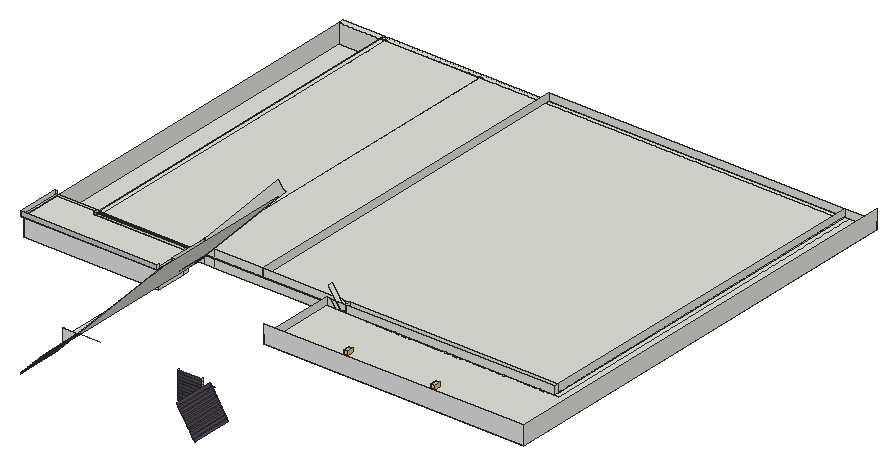
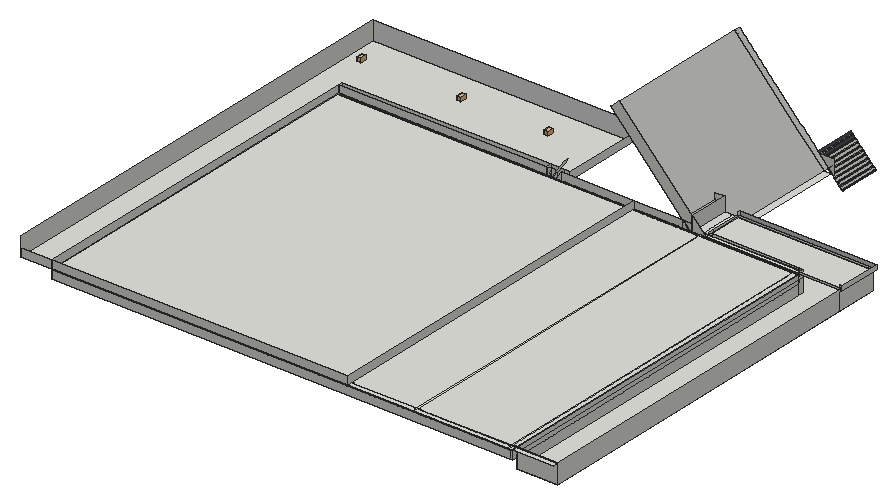
# SketchUp Ruby script. Lengths in inches.
U = 1.inch
M = Sketchup.active_model
def pt(a) = Geom::Point3d.new(a.map { |v| v * U })
def face(e, loops, mat)
  f = e.add_face(loops[0].map { |a| pt(a) })
  loops[1..].each { |l| e.add_face(l.map { |a| pt(a) }).erase! }
  f.material = f.back_material = mat if mat
  f
end
# faces: each face lists its corners as indices into pts; further lists are holes
def faces(e, pts, list, mat = nil) = list.each { |f| face(e, (f[0].is_a?(Array) ? f : [f]).map { |l| l.map { |i| pts[i] } }, mat) }
# xy, xz, yz: faces in a plane at the given z, y or x. An outline is a flat list of corners, or four numbers for a rectangle; further outlines are holes
def ring(l) = l.size == 4 ? [[l[0], l[1]], [l[2], l[1]], [l[2], l[3]], [l[0], l[3]]] : l.each_slice(2).to_a
def flat(e, list, mat, &to3) = list.each { |f| face(e, (f[0].is_a?(Array) ? f : [f]).map { |l| ring(l).map { |u, v| to3.(u, v) } }, mat) }
def xy(e, z, list, mat = nil) = flat(e, list, mat) { |x, y| [x, y, z] }
def xz(e, y, list, mat = nil) = flat(e, list, mat) { |x, z| [x, y, z] }
def yz(e, x, list, mat = nil) = flat(e, list, mat) { |y, z| [x, y, z] }
def lines(e, pts, list) = list.each { |a, b| e.add_line(pt(pts[a]), pt(pts[b])) }
# prism: a flat outline (further loops are holes) pulled along v
def prism(e, loops, v, mat = nil)
  f = face(e, loops, mat); d = Geom::Vector3d.new(v.map { |x| x * U })
  f.pushpull(f.normal.samedirection?(d) ? d.length : -d.length)
end
def box(e, o, s, mat = nil) = prism(e, [[o, [o[0] + s[0], o[1], o[2]], [o[0] + s[0], o[1] + s[1], o[2]], [o[0], o[1] + s[1], o[2]]]], [0, 0, s[2]], mat)
def at(x, y, z, deg = 0) = Geom::Transformation.translation(pt([x, y, z])) * Geom::Transformation.rotation(ORIGIN, Z_AXIS, deg.degrees)
def axes(o, x, y, z) = Geom::Transformation.new([*x, 0, *y, 0, *z, 0, *pt(o).to_a, 1])
def part(name) = M.definitions.add(name)
# library, detail: a bought-in or finely detailed component or shape, given as its bounding box
def library(name, o, s) = part(name).tap { |d| box(d.entities, o, s) }
def detail(e, o, s) = box(e.add_group.entities, o, s)
def put(e, d, t, mat = nil) = e.add_instance(d, t).tap { |i| i.material = mat if mat }
def group(e, t, mat = nil) = e.add_group.tap { |g| g.transformation = t; g.material = mat if mat }.entities
root = M.entities
M.materials.add("[Color M01]").color = [226, 226, 226]
M.materials.add("[Color M02]").color = [198, 198, 198]
M.materials.add("[Color M06]").color = [79, 71, 84]
c1 = library("Group\#13",[0,0,0],[3.54,3.54,3.9375])
xy(root,306.39,[[1096.79,2375.74,1127.76,2378.12]])
xy(root,307.2,[[1096.79,2375.74,1127.76,2378.12]])
xy(root,310.33,[[1096.79,2375.74,1127.76,2378.12]])
xy(root,311.14,[[1096.79,2375.74,1127.76,2378.12]])
xy(root,314.27,[[1096.79,2375.74,1127.76,2378.12]])
xy(root,315.08,[[1096.79,2376.24,1127.76,2378.12]])
xy(root,315.25,[[771.375,2530.63,771.375,3047.67,824.9375,3047.67,824.9375,2578.12,948.3125,2578.12,948.3125,2530.63]])
xy(root,318.2,[[1096.79,2376.24,1127.76,2378.12]])
xy(root,319.01,[[1096.79,2376.24,1127.76,2378.12]])
xy(root,322.14,[[1096.79,2376.24,1127.76,2378.12]])
xy(root,322.89,[[1096.79,2376.24,1127.76,2378.12]])
xy(root,326.02,[[1096.79,2376.24,1127.76,2378.12]])
xy(root,326.08,[[946.73,2380.48,955.23,2571.2],[946.73,2571.2,955.23,2571.59]])
xy(root,326.76,[[1096.79,2376.24,1127.76,2378.12]])
xy(root,328,[[824.9375,2584.2,1429.3,3053.87]])
xy(root,329.89,[[1096.79,2376.24,1127.76,2378.12]])
xy(root,330.64,[[1096.79,2376.24,1127.76,2378.12]])
xy(root,333.125,[[824.9375,2578.12,828.75,2584.2],[824.9375,2584.2,828.75,2586.43],[824.9375,2586.43,828.75,3047.67]])
xy(root,333.77,[[1096.79,2376.24,1127.76,2378.12]])
xy(root,334.51,[[1096.79,2376.24,1127.76,2378.12]])
xy(root,337.64,[[1096.79,2376.24,1127.76,2378.12]])
xy(root,338.39,[[1096.79,2376.24,1127.76,2378.12]])
xy(root,338.875,[[824.9375,2584.2,1429.3,3053.87]])
xy(root,340.125,[[1130.09,2475.84,1130.09,2578.12,1182.42,2578.12,1182.42,2576.81,1188.5,2576.81,1188.5,2578.12,1191.92,2578.12,1191.92,2576.81,1198,2576.81,1198,2578.12,1201.42,2578.12,1201.42,2576.81,1207.5,2576.81,1207.5,2578.12,1210.92,2578.12,1210.92,2576.81,1217,2576.81,1217,2578.12,1220.42,2578.12,1220.42,2576.81,1226.5,2576.81,1226.5,2578.12,1229.92,2578.12,1229.92,2576.81,1236,2576.81,1236,2578.12,1239.42,2578.12,1239.42,2576.81,1245.5,2576.81,1245.5,2578.12,1248.92,2578.12,1248.92,2576.81,1255,2576.81,1255,2578.12,1258.42,2578.12,1258.42,2576.81,1264.5,2576.81,1264.5,2578.12,1267.92,2578.12,1267.92,2576.81,1274,2576.81,1274,2578.12,1277.42,2578.12,1277.42,2576.81,1283.5,2576.81,1283.5,2578.12,1286.92,2578.12,1286.92,2576.81,1293,2576.81,1293,2578.12,1296.42,2578.12,1296.42,2576.81,1302.5,2576.81,1302.5,2578.12,1305.92,2578.12,1305.92,2576.81,1312,2576.81,1312,2578.12,1315.42,2578.12,1315.42,2576.81,1321.5,2576.81,1321.5,2578.12,1324.92,2578.12,1324.92,2576.81,1331,2576.81,1331,2578.12,1334.42,2578.12,1334.42,2576.81,1340.5,2576.81,1340.5,2578.12,1343.92,2578.12,1343.92,2576.81,1350,2576.81,1350,2578.12,1353.42,2578.12,1353.42,2576.81,1359.5,2576.81,1359.5,2578.12,1362.92,2578.12,1362.92,2576.81,1369,2576.81,1369,2578.12,1372.42,2578.12,1372.42,2576.81,1378.5,2576.81,1378.5,2578.12,1381.92,2578.12,1381.92,2576.81,1388,2576.81,1388,2578.12,1391.42,2578.12,1391.42,2576.81,1397.5,2576.81,1397.5,2578.12,1400.92,2578.12,1400.92,2576.81,1407,2576.81,1407,2578.12,1410.42,2578.12,1410.42,2576.81,1416.5,2576.81,1416.5,2578.12,1419.92,2578.12,1419.92,2576.81,1426,2576.81,1426,2578.12,1429.42,2578.12,1429.42,2576.81,1435.5,2576.81,1435.5,3053.87,1470.74,3053.87,1470.74,2475.84],[768.8125,2528.07,771.375,2530.63],[771.375,2528.07,948.3125,2530.63],[768.8125,2530.63,771.375,2584.2],[771.375,2530.63,771.375,2584.2,824.9375,2584.2,824.9375,2578.12,948.3125,2578.12,948.3125,2530.63],
  [948.3125,2530.63,954.51,2578.12],[954.51,2530.63,955.23,2578.12],[955.23,2530.63,965.61,2578.12],[965.61,2530.63,968.45,2578.12],[1182.42,2576.81,1188.5,2578.12],
  [1191.92,2576.81,1198,2578.12],[1201.42,2576.81,1207.5,2578.12],[1210.92,2576.81,1217,2578.12],[1220.42,2576.81,1226.5,2578.12],[1229.92,2576.81,1236,2578.12],
  [1239.42,2576.81,1245.5,2578.12],[1248.92,2576.81,1255,2578.12],[1258.42,2576.81,1264.5,2578.12],[1267.92,2576.81,1274,2578.12],[1277.42,2576.81,1283.5,2578.12],
  [1286.92,2576.81,1293,2578.12],[1296.42,2576.81,1302.5,2578.12],[1305.92,2576.81,1312,2578.12],[1315.42,2576.81,1321.5,2578.12],[1324.92,2576.81,1331,2578.12],
  [1334.42,2576.81,1340.5,2578.12],[1343.92,2576.81,1350,2578.12],[1353.42,2576.81,1359.5,2578.12],[1362.92,2576.81,1369,2578.12],[1372.42,2576.81,1378.5,2578.12],
  [1381.92,2576.81,1388,2578.12],[1391.42,2576.81,1397.5,2578.12],[1400.92,2576.81,1407,2578.12],[1410.42,2576.81,1416.5,2578.12],[1419.92,2576.81,1426,2578.12],
  [1429.42,2576.81,1435.5,3053.87],[824.9375,2578.12,831.01,2584.2],[831.01,2578.12,954.51,2584.2],[955.23,2578.12,965.61,2584.2],[965.61,2578.12,968.45,2584.2],
  [1156.15,2578.12,1429.3,2584.2],[1429.3,2578.12,1429.42,2584.2],[824.9375,2584.2,831.01,2586.43],[831.01,2584.2,954.51,2584.2,954.51,2584.32,831.14,2584.32,831.14,2586.43,831.01,2586.43],[954.51,2584.2,955.23,2586.43],
  [955.23,2584.2,1041.36,2586.43],[1041.36,2584.2,1156.15,2586.43],[1156.15,2584.2,1429.3,2586.43],[1429.3,2584.2,1429.42,2586.43],[831.14,2584.32,954.51,2586.43],
  [824.9375,2586.43,831.01,3047.67],[831.01,2586.43,831.14,3047.67],[831.14,2586.43,954.51,3047.67],[954.51,2586.43,955.23,3047.67],[955.23,2586.43,1041.36,3047.67],
  [1041.36,2586.43,1429.3,3047.67],[1429.3,2586.43,1429.42,3047.79],[771.375,3047.67,824.9375,3047.79],[824.9375,3047.67,828.75,3047.79],[828.75,3047.67,831.01,3047.79],
  [831.01,3047.67,954.51,3047.79],[954.51,3047.67,955.23,3047.79],[955.23,3047.67,1041.36,3047.79],[1041.36,3047.67,1429.3,3047.79],[771.375,3047.79,824.9375,3053.87],
  [824.9375,3047.79,828.75,3053.87],[828.75,3047.79,831.01,3053.87],[831.01,3047.79,954.51,3053.87],[954.51,3047.79,955.23,3053.87],[955.23,3047.79,1041.36,3053.87],
  [1041.36,3047.79,1429.3,3053.87],[1429.3,3047.79,1429.42,3053.87]])
xz(root,2373.56,[[1164.8,305.32,1165.17,305.56,1163.47,308.2,1163.11,307.97],[937.8,306.65,937.35,307.08,939.77,309.65,940.22,309.22],[937.35,307.08,937.12,307.29,939.54,309.87,939.77,309.65],[1162.57,308.8,1162.94,309.03,1161.25,311.68,1160.88,311.44],[941.1,310.16,940.64,310.59,943.07,313.16,943.52,312.73],
  [1160.35,312.27,1160.72,312.51,1159.02,315.15,1158.65,314.91],[944.4,313.66,943.94,314.09,946.36,316.66,946.82,316.23],[1158.12,315.74,1158.49,315.98,1156.8,318.62,1156.43,318.38],[947.7,317.17,947.24,317.59,948.3125,318.73,948.3125,317.82],[948.3125,317.82,948.77,318.3,948.3125,318.73],
  [948.77,318.3,950.12,319.74,949.66,320.17,948.3125,318.73],[948.3125,318.73,949.66,320.17,950.54,321.1,952.96,323.67,953.84,324.6,955.23,326.08,956.26,327.17,957.14,328.11,959.56,330.68,960.4375,331.61,962.86,334.18,963.73,335.11,966.16,337.6875,967.03,338.62,968.45,340.125,948.3125,340.125],[1155.9,319.21,1156.26,319.45,1154.57,322.09,1154.2,321.86],[951,320.67,953.42,323.24,952.96,323.67,950.54,321.1],[1153.67,322.6875,1154.04,322.92,1152.34,325.57,1151.98,325.33],
  [954.29,324.17,953.84,324.6,955.23,326.08,955.23,325.17],[955.23,325.17,955.6875,325.65,955.23,326.08],[955.6875,325.65,956.71,326.75,956.26,327.17,955.23,326.08],[1151.44,326.16,1151.8125,326.4,1150.12,329.04,1149.75,328.8],[957.59,327.68,960.01,330.25,959.56,330.68,957.14,328.11],
  [1149.22,329.63,1149.59,329.87,1147.89,332.51,1147.52,332.28],[960.89,331.18,963.3125,333.75,962.86,334.18,960.4375,331.61],[1146.99,333.11,1147.36,333.34,1145.66,335.98,1145.3,335.75],[964.1875,334.6875,966.61,337.26,966.16,337.6875,963.73,335.11],[1144.76,336.58,1145.13,336.8125,1143.4375,339.46,1143.07,339.22],
  [967.49,338.19,968.91,339.7,968.45,340.125,967.03,338.62],[968.91,339.7,969.31,340.125,968.45,340.125],[1142.54,340.05,1142.91,340.29,1141.21,342.93,1140.84,342.69],[968.45,340.125,969.31,340.125,969.91,340.76,969.45,341.19]])
xz(root,2375.74,[[1096.79,307.2,1127.76,310.33],[1096.79,311.14,1127.76,314.27]],"[Color M06]")
xz(root,2376.24,[[1096.79,315.08,1127.76,318.2],[1096.79,319.01,1127.76,322.14],[1096.79,322.89,1127.76,326.02],[1096.79,326.76,1127.76,329.89],[1096.79,330.64,1127.76,333.77],
  [1096.79,334.51,1127.76,337.64],[1096.79,338.39,1127.76,341.52]],"[Color M06]")
xz(root,2378.12,[[1096.79,306.39,1127.76,307.2],[1096.79,310.33,1127.76,311.14],[1096.79,314.27,1127.76,315.08],[1096.79,318.2,1127.76,319.01],[1096.79,322.14,1127.76,322.89],
  [1096.79,326.02,1127.76,326.76],[1096.79,329.89,1127.76,330.64],[1096.79,333.77,1127.76,334.51],[1096.79,337.64,1127.76,338.39]])
xz(root,2475.84,[[1130.09,340.125,1470.74,363.75]],"[Color M01]")
xz(root,2528.07,[[768.8125,340.125,948.3125,346.3125]],"[Color M02]")
xz(root,2530.63,[[771.375,340.125,948.3125,342.6875],[965.61,340.125,968.45,340.125,977.92,350.1875,977.92,358.5,965.61,358.5]])
xz(root,2530.63,[[771.375,315.25,948.3125,340.125]],"[Color M01]")
xz(root,2578.12,[[824.9375,315.25,828.75,333.125],[828.75,315.25,831.01,315.25,831.01,340.125,824.9375,340.125,824.9375,333.125,828.75,333.125],[831.01,315.25,943.125,340.125],[943.125,315.25,948.3125,340.125],[824.9375,340.125,831.01,342.6875],
  [831.01,340.125,943.125,342.6875],[943.125,340.125,948.3125,342.6875],[1130.09,340.125,1130.09,350.1875,1136.56,350.1875,1143.01,340.125],[1143.01,340.125,1148.73,340.125,1142.28,350.1875,1136.56,350.1875],[1148.73,340.125,1142.28,350.1875,1156.15,350.1875,1156.15,340.125,1153.99,343.5],
  [1148.73,340.125,1153.99,343.5,1156.15,340.125],[1156.15,340.125,1429.3,350.1875]])
xz(root,2583.74,[[955.23,326.08,944.56,336.13,948.3125,340.125,964.88,357.73,965.61,357.04,965.61,358.5,1061.61,460.49,1069.15,453.39,1072.29,450.4375,977.92,350.1875,968.45,340.125]])
xz(root,2584.2,[[955.23,326.08,955.23,328,957.04,328],[824.9375,328,831.01,338.875],[831.01,328,955.23,338.875],[955.23,328,955.23,338.875,965.61,338.875,965.61,337.11,957.04,328],[957.04,328,965.61,328,965.61,337.11],
  [965.61,328,977.92,328,977.92,338.875,967.27,338.875,965.61,337.11],[977.92,328,1136.56,338.875],[1136.56,328,1142.28,338.875],[1142.28,328,1149.7,328,1149.7,329.69,1143.8125,338.875,1142.28,338.875],[1149.7,328,1150.78,328,1149.7,329.69],
  [1150.78,328,1156.15,328,1156.15,338.875,1149.7,338.875,1149.7,329.69],[1156.15,328,1429.3,338.875],[1149.7,329.69,1149.7,338.875,1143.8125,338.875],[965.61,337.11,965.61,338.875,967.27,338.875],[824.9375,338.875,831.01,340.125],
  [831.01,338.875,955.23,340.125],[955.23,338.875,965.61,340.125],[965.61,338.875,965.61,340.125,968.45,340.125,967.27,338.875],[967.27,338.875,977.92,338.875,977.92,340.125,968.45,340.125],[977.92,338.875,1136.56,340.125],
  [1136.56,338.875,1142.28,340.125],[1142.28,338.875,1143.8125,338.875,1143.01,340.125,1142.28,340.125],[1143.8125,338.875,1149.7,338.875,1149.7,340.125,1143.01,340.125],[1149.7,338.875,1156.15,340.125],[1156.15,338.875,1429.3,340.125],
  [768.8125,340.125,771.375,346.3125],[771.375,340.125,824.9375,342.6875],[965.61,340.125,965.61,350.1875,977.92,350.1875,968.45,340.125],[968.45,340.125,977.92,350.1875,977.92,340.125],[977.92,340.125,1041.36,350.1875],
  [1041.36,340.125,1136.56,350.1875],[1136.56,340.125,1142.28,340.125,1142.28,341.27,1136.56,350.1875],[1142.28,340.125,1143.01,340.125,1142.28,341.27],[1143.01,340.125,1148.73,340.125,1142.28,350.1875,1142.28,341.27],[1148.73,340.125,1149.7,340.75,1149.7,350.1875,1142.28,350.1875],
  [1148.73,340.125,1149.7,340.125,1149.7,340.75],[1149.7,340.125,1156.15,340.125,1156.15,350.1875,1149.7,350.1875,1153.99,343.5,1149.7,340.75],[1156.15,340.125,1429.3,350.1875]])
xz(root,3047.67,[[771.375,315.25,824.9375,340.125],[824.9375,333.125,828.75,340.125]])
xz(root,3053.87,[[824.9375,328,828.75,338.875],[828.75,328,1429.3,338.875],[824.9375,338.875,828.75,340.125],[828.75,338.875,1429.3,340.125],[1041.36,340.125,1429.3,350.1875],
  [1429.3,340.125,1470.74,350.1875]])
yz(root,768.8125,[[2528.07,340.125,2584.2,346.3125]])
yz(root,771.375,[[2530.63,315.25,2584.2,340.125],[2584.2,315.25,3047.67,340.125],[2530.63,340.125,2584.2,342.6875]])
yz(root,824.9375,[[2578.12,315.25,2584.2,333.125],[2584.2,315.25,2586.43,328],[2586.43,315.25,3047.67,328],[2584.2,328,2586.43,333.125],[2586.43,328,3047.67,333.125],
  [3047.67,328,3053.87,338.875],[2578.12,333.125,2584.2,340.125],[2584.2,333.125,2586.43,338.875],[2586.43,333.125,3047.67,338.875],[2584.2,338.875,2586.43,340.125],
  [2586.43,338.875,3047.67,340.125],[3047.67,338.875,3053.87,340.125],[2578.12,340.125,2584.2,342.6875]])
yz(root,948.3125,[[2530.63,315.25,2571.59,340.125],[2571.59,315.25,2578.12,340.125],[2528.07,340.125,2530.63,346.3125],[2530.63,340.125,2571.59,342.6875],[2571.59,340.125,2578.12,342.6875]])
yz(root,955.23,[[2578.12,326.08,2584.2,340.125]])
yz(root,965.61,[[2530.63,340.125,2583.74,358.5],[2583.74,340.125,2584.2,358.5]])
yz(root,1041.36,[[2584.2,340.125,3053.87,350.1875]])
yz(root,1096.79,[[2375.74,307.2,2378.12,310.33],[2375.74,311.14,2378.12,314.27],[2376.24,315.08,2378.12,318.2],[2376.24,319.01,2378.12,322.14],[2376.24,322.89,2378.12,326.02],
  [2376.24,326.76,2378.12,329.89],[2376.24,330.64,2378.12,333.77],[2376.24,334.51,2378.12,337.64],[2376.24,338.39,2378.12,341.52]])
yz(root,1127.76,[[2375.74,307.2,2378.12,310.33],[2375.74,311.14,2378.12,314.27],[2376.24,315.08,2378.12,318.2],[2376.24,319.01,2378.12,322.14],[2376.24,322.89,2378.12,326.02],
  [2376.24,326.76,2378.12,329.89],[2376.24,330.64,2378.12,333.77],[2376.24,334.51,2378.12,337.64],[2376.24,338.39,2378.12,341.52]])
yz(root,1130.09,[[2475.84,340.125,2578.12,350.1875]])
yz(root,1156.15,[[2578.12,340.125,2584.2,350.1875]])
yz(root,1429.3,[[2584.2,328,3047.67,338.875],[3047.67,328,3053.87,338.875],[2584.2,338.875,3047.67,340.125],[3047.67,338.875,3053.87,340.125],[2578.12,340.125,2584.2,350.1875],
  [2584.2,340.125,3053.87,350.1875]])
yz(root,1470.74,[[2475.84,340.125,3053.87,363.75]])
p = [[1163.11,2373.56,307.97],[1164.8,2373.56,305.32],[1164.8,2319.18,305.32],[1163.11,2319.18,307.97],[1165.17,2373.56,305.56],[1165.17,2319.18,305.56],
  [936.47,2373.56,306.15],[936.47,2319.18,306.15],[936.92,2319.18,305.72],[936.92,2373.56,305.72],[936.24,2373.56,306.36],[936.24,2319.18,306.36],
  [937.35,2373.56,307.08],[937.35,2319.18,307.08],[937.8,2373.56,306.65],[937.8,2319.18,306.65],[940.22,2373.56,309.22],[940.22,2319.18,309.22],
  [937.12,2319.18,307.29],[937.12,2373.56,307.29],[939.77,2373.56,309.65],[939.77,2319.18,309.65],[939.54,2373.56,309.87],[939.54,2319.18,309.87],
  [1163.47,2319.18,308.2],[1163.47,2373.56,308.2],[1162.94,2319.18,309.03],[1162.94,2373.56,309.03],[1160.88,2373.56,311.44],[1162.57,2373.56,308.8],
  [1162.57,2319.18,308.8],[1160.88,2319.18,311.44],[940.64,2373.56,310.59],[940.64,2319.18,310.59],[941.1,2373.56,310.16],[941.1,2319.18,310.16],
  [943.52,2373.56,312.73],[943.52,2319.18,312.73],[943.07,2373.56,313.16],[943.07,2319.18,313.16],[1161.25,2319.18,311.68],[1161.25,2373.56,311.68],
  [1160.72,2319.18,312.51],[1160.72,2373.56,312.51],[1158.65,2373.56,314.91],[1160.35,2373.56,312.27],[1160.35,2319.18,312.27],[1158.65,2319.18,314.91],
  [943.94,2373.56,314.09],[943.94,2319.18,314.09],[944.4,2373.56,313.66],[944.4,2319.18,313.66],[946.82,2373.56,316.23],[946.82,2319.18,316.23],
  [946.36,2373.56,316.66],[946.36,2319.18,316.66],[1159.02,2319.18,315.15],[1159.02,2373.56,315.15],[1158.49,2319.18,315.98],[1158.49,2373.56,315.98],
  [1156.43,2373.56,318.38],[1158.12,2373.56,315.74],[1158.12,2319.18,315.74],[1156.43,2319.18,318.38],[947.24,2373.56,317.59],[947.24,2319.18,317.59],
  [947.7,2373.56,317.17],[947.7,2319.18,317.17],[948.77,2373.56,318.3],[950.12,2373.56,319.74],[950.12,2319.18,319.74],[948.3125,2373.56,317.82],
  [949.66,2373.56,320.17],[948.3125,2373.56,318.73],[949.66,2319.18,320.17],[1156.8,2319.18,318.62],[1156.8,2373.56,318.62],[1156.26,2319.18,319.45],
  [1156.26,2373.56,319.45],[1154.2,2373.56,321.86],[1155.9,2373.56,319.21],[1155.9,2319.18,319.21],[1154.2,2319.18,321.86],[950.54,2373.56,321.1],
  [950.54,2319.18,321.1],[951,2373.56,320.67],[951,2319.18,320.67],[953.42,2373.56,323.24],[953.42,2319.18,323.24],[952.96,2373.56,323.67],
  [952.96,2319.18,323.67],[1154.57,2319.18,322.09],[1154.57,2373.56,322.09],[1154.04,2319.18,322.92],[1154.04,2373.56,322.92],[1151.98,2373.56,325.33],
  [1153.67,2373.56,322.6875],[1153.67,2319.18,322.6875],[1151.98,2319.18,325.33],[953.84,2373.56,324.6],[953.84,2319.18,324.6],[954.29,2373.56,324.17],
  [954.29,2319.18,324.17],[955.6875,2373.56,325.65],[956.71,2373.56,326.75],[956.71,2319.18,326.75],[955.23,2373.56,325.17],[956.26,2373.56,327.17],
  [955.23,2373.56,326.08],[956.26,2319.18,327.17],[1152.34,2319.18,325.57],[1152.34,2373.56,325.57],[1151.8125,2319.18,326.4],[1151.8125,2373.56,326.4],
  [955.23,2380.48,326.08],[1072.29,2380.48,450.4375],[1072.29,2373.56,450.4375],[1071.98,2373.56,450.11],[1071.71,2373.56,449.82],[1069.29,2373.56,447.25],
  [1068.41,2373.56,446.32],[1065.99,2373.56,443.75],[1065.11,2373.56,442.8125],[1062.69,2373.56,440.24],[1061.8125,2373.56,439.31],[1059.39,2373.56,436.74],
  [1058.51,2373.56,435.81],[1056.09,2373.56,433.23],[1055.22,2373.56,432.3],[1052.79,2373.56,429.73],[1051.92,2373.56,428.8],[1049.5,2373.56,426.23],
  [1048.62,2373.56,425.29],[1046.2,2373.56,422.72],[1045.32,2373.56,421.79],[1042.9,2373.56,419.22],[1042.02,2373.56,418.28],[1039.6,2373.56,415.71],
  [1038.72,2373.56,414.78],[1036.3,2373.56,412.21],[1035.42,2373.56,411.28],[1033,2373.56,408.7],[1032.125,2373.56,407.77],[1029.71,2373.56,405.2],
  [1028.83,2373.56,404.27],[1026.41,2373.56,401.7],[1025.53,2373.56,400.76],[1023.11,2373.56,398.19],[1022.23,2373.56,397.26],[1019.81,2373.56,394.6875],
  [1018.93,2373.56,393.75],[1016.51,2373.56,391.18],[1015.63,2373.56,390.25],[1013.21,2373.56,387.68],[1012.33,2373.56,386.75],[1009.91,2373.56,384.17],
  [1009.04,2373.56,383.24],[1006.62,2373.56,380.67],[1005.74,2373.56,379.74],[1003.32,2373.56,377.17],[1002.4375,2373.56,376.23],[1000.02,2373.56,373.66],
  [999.14,2373.56,372.73],[996.72,2373.56,370.16],[995.84,2373.56,369.23],[993.42,2373.56,366.65],[992.54,2373.56,365.72],[990.12,2373.56,363.15],
  [989.25,2373.56,362.22],[986.82,2373.56,359.64],[985.95,2373.56,358.71],[983.53,2373.56,356.14],[982.65,2373.56,355.21],[980.23,2373.56,352.64],
  [979.35,2373.56,351.7],[976.93,2373.56,349.13],[976.05,2373.56,348.2],[973.63,2373.56,345.63],[972.75,2373.56,344.7],[970.33,2373.56,342.125],
  [969.45,2373.56,341.19],[968.45,2373.56,340.125],[967.03,2373.56,338.62],[966.16,2373.56,337.6875],[963.73,2373.56,335.11],[962.86,2373.56,334.18],
  [960.4375,2373.56,331.61],[959.56,2373.56,330.68],[957.14,2373.56,328.11],[955.23,2571.59,326.08],[968.45,2571.59,340.125],[968.45,2530.63,340.125],
  [977.92,2530.63,350.1875],[977.92,2571.59,350.1875],[1072.29,2571.59,450.4375],[955.23,2571.2,326.08],[944.56,2571.2,336.13],[944.56,2583.74,336.13],
  [955.23,2583.74,326.08],[955.23,2578.12,326.08],[968.45,2578.12,340.125],[968.45,2583.74,340.125],[968.45,2584.2,340.125],[967.27,2584.2,338.875],
  [965.61,2584.2,337.11],[957.04,2584.2,328],[955.23,2584.2,326.08],[1149.75,2373.56,328.8],[1151.44,2373.56,326.16],[1151.44,2319.18,326.16],
  [1149.75,2319.18,328.8],[957.14,2319.18,328.11],[957.59,2373.56,327.68],[957.59,2319.18,327.68],[960.01,2373.56,330.25],[960.01,2319.18,330.25],
  [959.56,2319.18,330.68],[1150.12,2319.18,329.04],[1150.12,2373.56,329.04],[1149.59,2319.18,329.87],[1149.59,2373.56,329.87],[1147.52,2373.56,332.28],
  [1149.22,2373.56,329.63],[1149.22,2319.18,329.63],[1147.52,2319.18,332.28],[960.4375,2319.18,331.61],[960.89,2373.56,331.18],[960.89,2319.18,331.18],
  [963.3125,2373.56,333.75],[963.3125,2319.18,333.75],[962.86,2319.18,334.18],[1147.89,2319.18,332.51],[1147.89,2373.56,332.51],[1147.36,2319.18,333.34],
  [1147.36,2373.56,333.34],[1145.3,2373.56,335.75],[1146.99,2373.56,333.11],[1146.99,2319.18,333.11],[1145.3,2319.18,335.75],[963.73,2319.18,335.11],
  [964.1875,2373.56,334.6875],[964.1875,2319.18,334.6875],[966.61,2373.56,337.26],[966.61,2319.18,337.26],[1145.66,2319.18,335.98],[1145.66,2373.56,335.98],
  [1145.13,2319.18,336.8125],[1145.13,2373.56,336.8125],[1143.07,2373.56,339.22],[1144.76,2373.56,336.58],[1144.76,2319.18,336.58],[1143.07,2319.18,339.22],
  [966.16,2319.18,337.6875],[967.03,2319.18,338.62],[967.49,2373.56,338.19],[967.49,2319.18,338.19],[969.31,2373.56,340.125],[969.91,2373.56,340.76],
  [969.91,2319.18,340.76],[968.91,2373.56,339.7],[1143.4375,2319.18,339.46],[1143.4375,2373.56,339.46],[1142.91,2319.18,340.29],[1142.91,2373.56,340.29],
  [1143.01,2373.56,340.125],[1140.84,2373.56,342.69],[1142.54,2373.56,340.05],[1142.54,2319.18,340.05],[1140.84,2319.18,342.69],[977.92,2583.74,350.1875],
  [1133.58,2578.12,363.75],[1132.82,2578.12,364.9375],[1132.82,2584.2,364.9375],[1142.28,2584.2,350.1875],[1148.73,2584.2,340.125],[1148.73,2578.12,340.125],
  [1142.28,2578.12,350.1875],[1136.56,2578.12,359.1],[1153.99,2578.12,343.5],[1149.7,2584.2,340.75],[1153.99,2584.2,343.5],[977.92,2584.2,350.1875],
  [944.56,2380.48,336.13],[948.3125,2578.12,340.125],[948.3125,2583.74,340.125],[997.28,2373.56,340.125],[1148.73,2373.56,340.125]]
faces(root,p,[[0,1,2,3],[6,12,13,7],[13,12,14,15],[14,16,17,15],[24,26,27,25],[28,29,30,31],[20,32,33,21],[33,32,34,35],
  [34,36,37,35],[40,42,43,41],[44,45,46,47],[38,48,49,39],[50,52,53,51],[56,58,59,57],[60,61,62,63],[54,64,65,55],
  [68,69,70,67,66,71],[75,77,78,76],[79,80,81,82],[72,83,84,74],[85,87,88,86],[91,93,94,92],[95,96,97,98],[89,99,100,90],
  [103,104,105,102,101,106],[110,112,113,111],[207,208,209,210],[107,188,211,109],[212,214,215,213],[217,219,220,218],[221,222,223,224],[187,186,225,216],
  [226,228,229,227],[231,233,234,232],[235,236,237,238],[185,184,239,230],[240,242,243,241],[244,246,247,245],[248,249,250,251],[183,182,253,252],
  [256,257,258,255,254,259],[260,262,263,264,261],[265,266,267,268]],"[Color M06]")
faces(root,p,[[4,5,2,1],[6,7,8,9],[7,6,10,11],[12,13,18,19],[20,12,13,21],[22,19,18,23],[24,25,0,3],[27,26,30,29],
  [20,21,17,16],[21,20,22,23],[38,32,33,39],[40,41,28,31],[43,42,46,45],[38,39,37,36],[49,48,50,51],[54,48,49,55],
  [56,57,44,47],[59,58,62,61],[54,55,53,52],[65,64,66,67],[72,73,64,65,74],[75,76,60,63],[78,77,81,80],[72,74,70,69],
  [84,83,85,86],[89,83,84,90],[91,92,79,82],[94,93,97,96],[89,90,88,87],[100,99,101,102],[107,108,99,100,109],[110,111,95,98],
  [114,115,116,117,118,119,120,121,122,123,124,125,126,127,128,129,130,131,132,133,134,135,136,137,138,139,140,141,142,143,144,145,146,147,148,149,150,151,152,153,154,155,156,157,158,159,160,161,162,163,164,165,166,167,168,169,170,171,172,173,174,175,176,177,178,179,180,181,182,183,184,185,186,187,188,107,108],[189,190,191,192,193,194,115,114,195],[189,195,196,197,198,199],[189,190,200,201,198,199],[198,201,202,203,204,205,206],[113,112,209,208],[107,109,105,104],[211,188,212,213],
  [187,188,211,216],[217,218,207,210],[220,219,223,222],[187,216,215,214],[225,186,226,227],[185,186,225,230],[231,232,221,224],[234,233,237,236],
  [185,230,229,228],[239,184,240,241],[244,245,235,238],[247,246,250,249],[183,252,243,242],[253,182,254,255],[260,261,248,251],[263,262,267,266],
  [190,193,192,191],[190,193,269,201,200],[270,271,272,273,274,275,276,277],[278,275,274,279,280],[269,201,202,281]])
lines(root,p,[[114,282],[283,284],[285,256],[264,286]])
put(root,c1,axes([1326.69,2510.51,344.6875],[-1.5535,0,0],[0,2.39,0],[0,0,-3.63878]))
put(root,c1,axes([1212.13,2510.51,344.6875],[-1.5535,0,0],[0,2.39,0],[0,0,-3.63878]))
put(root,c1,axes([1457.26,2510.51,344.6875],[-1.5535,0,0],[0,2.39,0],[0,0,-3.63878]))
